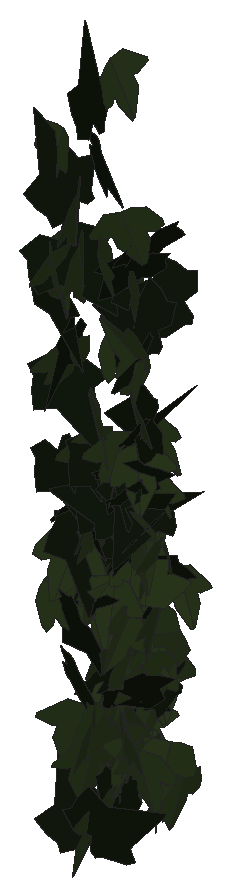
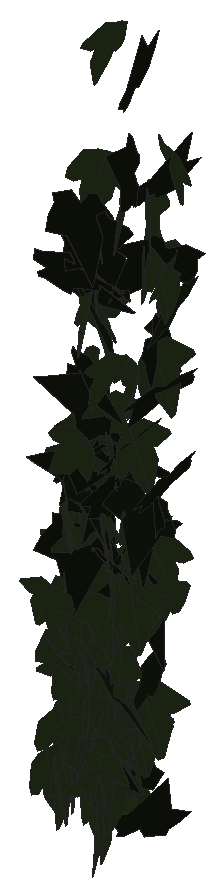
# SketchUp Ruby script. Lengths in inches.
U = 1.inch
M = Sketchup.active_model
def pt(a) = Geom::Point3d.new(a.map { |v| v * U })
def face(e, loops, mat)
  f = e.add_face(loops[0].map { |a| pt(a) })
  loops[1..].each { |l| e.add_face(l.map { |a| pt(a) }).erase! }
  f.material = f.back_material = mat if mat
  f
end
# faces: each face lists its corners as indices into pts; further lists are holes
def faces(e, pts, list, mat = nil) = list.each { |f| face(e, (f[0].is_a?(Array) ? f : [f]).map { |l| l.map { |i| pts[i] } }, mat) }
# xy, xz, yz: faces in a plane at the given z, y or x. An outline is a flat list of corners, or four numbers for a rectangle; further outlines are holes
def ring(l) = l.size == 4 ? [[l[0], l[1]], [l[2], l[1]], [l[2], l[3]], [l[0], l[3]]] : l.each_slice(2).to_a
def flat(e, list, mat, &to3) = list.each { |f| face(e, (f[0].is_a?(Array) ? f : [f]).map { |l| ring(l).map { |u, v| to3.(u, v) } }, mat) }
def xy(e, z, list, mat = nil) = flat(e, list, mat) { |x, y| [x, y, z] }
def xz(e, y, list, mat = nil) = flat(e, list, mat) { |x, z| [x, y, z] }
def yz(e, x, list, mat = nil) = flat(e, list, mat) { |y, z| [x, y, z] }
def lines(e, pts, list) = list.each { |a, b| e.add_line(pt(pts[a]), pt(pts[b])) }
# prism: a flat outline (further loops are holes) pulled along v
def prism(e, loops, v, mat = nil)
  f = face(e, loops, mat); d = Geom::Vector3d.new(v.map { |x| x * U })
  f.pushpull(f.normal.samedirection?(d) ? d.length : -d.length)
end
def box(e, o, s, mat = nil) = prism(e, [[o, [o[0] + s[0], o[1], o[2]], [o[0] + s[0], o[1] + s[1], o[2]], [o[0], o[1] + s[1], o[2]]]], [0, 0, s[2]], mat)
def at(x, y, z, deg = 0) = Geom::Transformation.translation(pt([x, y, z])) * Geom::Transformation.rotation(ORIGIN, Z_AXIS, deg.degrees)
def axes(o, x, y, z) = Geom::Transformation.new([*x, 0, *y, 0, *z, 0, *pt(o).to_a, 1])
def part(name) = M.definitions.add(name)
# library, detail: a bought-in or finely detailed component or shape, given as its bounding box
def library(name, o, s) = part(name).tap { |d| box(d.entities, o, s) }
def detail(e, o, s) = box(e.add_group.entities, o, s)
def put(e, d, t, mat = nil) = e.add_instance(d, t).tap { |i| i.material = mat if mat }
def group(e, t, mat = nil) = e.add_group.tap { |g| g.transformation = t; g.material = mat if mat }.entities
root = M.entities
M.materials.add("efeu1").color = [18, 25, 13]
M.materials.add("efeu2").color = [43, 57, 29]
c1 = part("ivyleaf_9")
p = [[1.54,2.16,1.25],[1.36,2.04,1.19],[-0.21,0.99,0.68],[-0.71,1.11,0.82],[-0.85,0.86,0.67],[-0.8,0.17,0.21],
  [-0.9,-0.01,0.1],[-0.67,-0.16,-0.02],[-0.08,-0.08,-0.05],[-0.03,-0.6,-0.4],[0.65,-0.88,-0.66],[0.83,-0.6,-0.49],
  [1.29,-0.42,-0.43],[1.8125,-0.07,-0.26],[1.21,0.44,0.15]]
faces(c1.entities,p,[[0,1,2,3,4,5,6,7,8,9,10,11,12,13,14]],"efeu1")
c2 = part("ivyleaf_10")
p = [[0,0.5,-0.03],[-0.0625,2.02,-0.43],[-0.19,2.01,-0.46],[-0.54,1.05,-0.29],[-0.52,0.625,-0.18],[-0.83,0.76,-0.28],
  [-1.16,0.64,-0.33],[-1.15,0.33,-0.24],[-0.77,-0.39,0.02],[-0.3,-0.51,0.16],[0.04,-0.48,0.23],[-0.02,2.01,-0.4375],
  [-0.06,2.01,-0.43],[0.04,-0.49,0.23],[0.67,-0.49,0.14],[1.38,0.36,-0.2],[1.375,0.51,-0.24],[0.81,0.65,-0.19],
  [0.62,0.59,-0.15],[0.6,1.09,-0.28],[0.5,1.23,-0.31]]
faces(c2.entities,p,[[0,1,2,3,4,5,6,7,8,9,10],[11,12,0,13,14,15,16,17,18,19,20]],"efeu2")
put(root,c1,axes([503.85,135.93,193.72],[0.29247,-0.67636,-0.23949],[-0.06673,0.23186,-0.73631],[0.7144,0.29856,0.02927]))
put(root,c2,axes([504.13,135.48,202.97],[0.65071,-0.36372,0.02117],[0.02149,-0.00643,-0.73192],[0.39285,0.60282,0.00497]))
put(root,c2,axes([504.11,135.52,199.69],[-0.29868,0.74738,-0.07122],[0.01965,-0.06884,-0.80482],[-0.75051,-0.29924,0.00727]))
put(root,c2,axes([504.05,135.49,190.06],[0.08819,0.63214,0.37363],[0.04455,0.35691,-0.66288],[-0.784,0.09138,0.00436]))
put(root,c2,axes([504.33,135.49,199.79],[-0.02818,-0.80038,-0.11798],[-0.0198,0.11869,-0.80053],[0.80879,-0.02498,-0.02371]))
put(root,c2,axes([504.36,135.71,196.93],[-0.09748,-0.77423,0.14032],[-0.03583,-0.13688,-0.78013],[0.78602,-0.10226,-0.01816]))
put(root,c1,axes([503.82,135.64,198.59],[0.40294,-0.67919,0.14319],[0.07626,-0.12125,-0.78971],[0.68992,0.41008,0.00366]))
put(root,c1,axes([504.55,136.12,183.22],[-0.54458,-0.44797,0.2202],[0.19318,0.11714,0.70079],[-0.49904,0.5342,0.03098]))
put(root,c2,axes([504.46,136.59,190.1875],[-0.26662,-0.69959,0.04964],[0.01187,-0.0576,-0.74801],[0.70125,-0.26501,0.03153]))
put(root,c1,axes([504.57,135.91,192.6875],[0.16065,0.67425,0.16954],[-0.05888,0.17758,-0.71209],[-0.74686,0.13103,0.09261]))
put(root,c1,axes([504.06,135.82,196.26],[0.19336,-0.71103,-0.28018],[0.06705,0.30368,-0.72439],[0.7613,0.15385,0.13496]))
put(root,c1,axes([504.7,135.33,201.68],[-0.32899,-0.68329,0.30857],[0.1248,0.28235,0.75831],[-0.73928,0.35174,-0.0093]))
put(root,c2,axes([504.45,135.7,191.39],[0.73109,0.20015,-0.15467],[-0.15667,-0.03386,-0.73409],[-0.21904,0.69226,0.00881]))
put(root,c1,axes([504.35,135.73,187.875],[0.57329,-0.21264,-0.36386],[-0.32972,0.17613,-0.59305],[0.29463,0.61087,0.04433]))
put(root,c1,axes([504.71,135.71,192.4],[0.42549,0.08154,-0.57527],[-0.60291,0.01959,-0.41051],[-0.03371,0.67882,0.08095]))
put(root,c2,axes([504.79,135.7,186.67],[-0.54553,-0.51842,0.24353],[-0.14596,-0.19939,-0.7514],[0.55386,-0.56316,0.04185]))
put(root,c1,axes([504.49,135.67,197.51],[-0.20411,0.17828,-0.66152],[0.50675,-0.42947,-0.27017],[-0.50219,-0.50583,-0.00376]))
put(root,c1,axes([505.07,136.51,185.14],[-0.17766,0.29629,0.61295],[-0.30257,0.51855,-0.35243],[-0.645,-0.32486,-0.00351]))
put(root,c1,axes([504.26,135.5,200.09],[0.00591,-0.44392,-0.67778],[0.222,0.65274,-0.42559],[0.77921,-0.1826,0.1264]))
put(root,c1,axes([505.06,136.83,187.7],[-0.53617,0.43246,0.0549],[-0.04682,0.0306,-0.68471],[-0.46819,-0.49832,0.0056]))
put(root,c2,axes([504.64,136,191.47],[0.23655,-0.57216,0.31831],[-0.12167,0.2846,0.63715],[-0.69014,-0.24629,-0.00323]))
put(root,c2,axes([504.72,136.72,188.32],[0.11736,-0.65889,-0.32619],[0.00512,0.33104,-0.66685],[0.7352,0.10287,0.05671]))
put(root,c2,axes([504.79,136.9,184.89],[-0.09356,-0.66841,-0.24276],[0.04432,0.2389,-0.67485],[0.70975,-0.10303,0.01014]))
put(root,c2,axes([504.8,135.375,201.47],[0.27227,-0.72391,-0.265],[-0.0089,0.27807,-0.76877],[0.77084,0.25891,0.08472]))
put(root,c1,axes([504.52,136.09,191.7],[0.01968,-0.76216,-0.05621],[-0.00299,0.05615,-0.76241],[0.76423,0.01985,-0.00153]))
put(root,c2,axes([504.83,136.62,190.23],[0.14349,-0.65581,-0.33627],[0.01404,0.34496,-0.66675],[0.73686,0.12114,0.07819]))
put(root,c1,axes([505.2,135.09,189.75],[0.25131,0.19547,-0.76499],[-0.777,-0.08144,-0.27606],[-0.14031,0.80108,0.1586]))
put(root,c2,axes([504.84,136.6,190.38],[0.1255,-0.71483,-0.19602],[0.00745,0.20002,-0.72463],[0.74118,0.11903,0.04047]))
put(root,c2,axes([504.9,135.97,194.43],[-0.08873,-0.75427,0.18352],[0.0204,-0.18692,-0.75836],[0.776,-0.08133,0.04092]))
put(root,c2,axes([504.96,137.09,184.1],[0.14571,-0.58366,-0.38437],[-0.06892,0.37872,-0.60121],[0.69545,0.15982,0.02095]))
put(root,c2,axes([504.9,137.43,183.88],[0.3272,-0.56485,-0.26269],[0.036,0.31337,-0.62898],[0.6219,0.27904,0.17461]))
put(root,c2,axes([504.99,136.02,192.12],[0.13697,-0.67875,-0.32838],[0.03072,0.3385,-0.68686],[0.75339,0.10959,0.08771]))
put(root,c2,axes([505.01,135.22,200.06],[0.27493,-0.71871,-0.2534],[0.07213,0.29272,-0.75197],[0.75866,0.23262,0.16333]))
put(root,c2,axes([505.16,135.59,185.85],[-0.22808,-0.69401,0.0999],[-0.0223,-0.09782,-0.73047],[0.70081,-0.22898,0.00927]))
put(root,c2,axes([505.05,137.21,184.8125],[0.45925,-0.54338,-0.06754],[0.00247,0.09021,-0.70894],[0.54755,0.45534,0.05985]))
put(root,c2,axes([505.23,135.43,186.54],[0.20366,-0.64066,-0.42388],[-0.0688,0.42155,-0.67019],[0.7651,0.20844,0.05256]))
put(root,c1,axes([505.59,136.39,190.89],[-0.71501,0.20383,0.05754],[-0.06368,-0.00355,-0.7201],[-0.21904,-0.66435,0.0215]))
put(root,c2,axes([505.08,137.16,184.9375],[0.2397,0.67519,0.06414],[-0.02972,0.07841,-0.71444],[-0.67758,0.23542,0.05402]))
put(root,c2,axes([505.07,136.6,196.92],[0.0239,0.5762,0.30791],[0.02519,0.29534,-0.59958],[-0.69918,0.03033,-0.01108]))
put(root,c2,axes([505.01,136.88,186.875],[0.61212,0.3818,0.10176],[0.06428,0.08892,-0.72027],[-0.38987,0.61412,0.04102]))
put(root,c2,axes([505.37,136.98,185.8125],[-0.18151,-0.41509,0.5609],[-0.11951,-0.55251,-0.44755],[0.68747,-0.20564,0.07029]))
put(root,c2,axes([505.04,137.17,185.39],[0.65485,0.27704,0.11574],[0.09951,0.06173,-0.71082],[-0.28327,0.66213,0.01785]))
put(root,c1,axes([504.72,136.26,202.5625],[0.19608,-0.05369,-0.67659],[0.70177,-0.04966,0.19285],[-0.06736,-0.6736,0.03972]))
put(root,c2,axes([505.24,135.73,183.92],[0.21221,-0.65109,0.3794],[0.09858,-0.36678,-0.68457],[0.74709,0.23334,-0.01744]))
put(root,c2,axes([505.32,137.26,184.47],[0.14229,-0.6955,0.01762],[0.02136,-0.01361,-0.70967],[0.6954,0.14273,0.01819]))
put(root,c2,axes([505.38,137.17,184.2],[0.4199,-0.55474,-0.16486],[-0.05463,0.16478,-0.69361],[0.57613,0.41993,0.05439]))
put(root,c1,axes([505.05,135.88,194.29],[0.25686,-0.70449,-0.20401],[-0.02539,0.20749,-0.74847],[0.733,0.25406,0.04556]))
put(root,c2,axes([505.41,136.75,187.11],[-0.34813,-0.62884,-0.16639],[0.10716,0.13069,-0.71816],[0.64159,-0.36304,0.02967]))
put(root,c1,axes([505.61,135.05,204.34],[-0.10083,-0.50517,0.65479],[0.13692,0.64033,0.5151],[-0.81559,0.16995,0.00552]))
put(root,c2,axes([505.43,137.02,185.69],[0.68319,0.19789,-0.13654],[-0.13545,-0.023,-0.71111],[-0.19864,0.69632,0.01531]))
put(root,c2,axes([505.41,136.69,189.56],[-0.72112,-0.02035,-0.16316],[0.16434,-0.06539,-0.71817],[0.00534,-0.73645,0.06828]))
put(root,c1,axes([505.21,136.13,193.21],[0.17575,-0.63052,-0.48216],[-0.08503,0.47604,-0.65351],[0.78918,0.19171,0.03696]))
put(root,c2,axes([505.49,136.45,191.8],[0.39405,-0.64188,-0.09922],[0.01309,0.12387,-0.74941],[0.64937,0.38701,0.07531]))
put(root,c2,axes([505.42,135.42,195.79],[-0.49829,0.56556,-0.12774],[0.05894,-0.11386,-0.75847],[-0.62226,-0.46367,0.03045]))
put(root,c2,axes([505.68,136.96,198.64],[-0.41799,0.36555,0.34872],[-0.24734,0.24557,-0.55335],[-0.47521,-0.44935,-0.01872]))
put(root,c2,axes([505.6,136.0625,194.02],[0.45016,-0.63597,-0.24936],[-0.08748,0.2425,-0.77641],[0.67748,0.45389,0.06543]))
put(root,c2,axes([505.52,136.5,186.58],[-0.42623,0.61962,0.01152],[-0.00791,0.00855,-0.75207],[-0.61968,-0.4263,0.00167]))
put(root,c2,axes([505.58,136.47,186.91],[-0.00479,-0.64637,-0.35972],[0.09243,0.35638,-0.6416],[0.73392,-0.0491,0.07846]))
put(root,c2,axes([506.09,136.98,185.37],[-0.01324,0.02492,-0.63066],[-0.65496,0.02342,0.01375],[0.02586,0.60608,0.0254]))
put(root,c2,axes([505.67,136.17,184.63],[-0.04849,-0.71919,-0.11963],[0.02509,0.11817,-0.72062],[0.72864,-0.05193,0.01685]))
put(root,c1,axes([506.09,135.67,184.37],[-0.07312,0.16088,0.66524],[-0.4149,0.51307,-0.1765],[-0.57904,-0.38794,0.04246]))
put(root,c2,axes([505.8125,135.97,190.22],[-0.45941,-0.51113,0.3166],[-0.09837,-0.32918,-0.67418],[0.59314,-0.45048,0.13341]))
put(root,c2,axes([505.75,135.9,185.09],[0.45415,-0.45244,-0.34408],[-0.10902,0.36291,-0.62109],[0.55787,0.43925,0.15874]))
put(root,c1,axes([506.32,135.36,193.32],[-0.43687,0.13189,0.5506],[-0.5481,0.15102,-0.4424],[-0.21634,-0.64893,0.00896]))
put(root,c2,axes([505.42,136.5625,184.09],[-0.2791,0.20552,-0.62921],[0.33724,-0.54344,-0.32709],[-0.56958,-0.42247,0.11465]))
put(root,c2,axes([505.72,135.55,187.01],[-0.03496,-0.55942,-0.56628],[0.12688,0.55567,-0.55677],[0.78583,-0.1146,0.0647]))
put(root,c2,axes([505.54,136.92,186.24],[0.30527,0.61406,0.24078],[0.11036,0.21402,-0.68575],[-0.65028,0.32459,-0.00335]))
put(root,c2,axes([505.78,136.7,187.88],[0.32467,-0.62627,-0.21445],[0.01632,0.24636,-0.69473],[0.66176,0.30118,0.12235]))
put(root,c2,axes([505.87,136.1875,188.24],[-0.00982,0.65143,-0.34534],[-0.1261,-0.34176,-0.6411],[-0.72644,0.05052,0.11596]))
put(root,c2,axes([505.76,135.63,190.57],[0.75117,0.04653,0.05442],[0.05644,0.00271,-0.72496],[-0.05033,0.69749,-0.00082]))
put(root,c2,axes([506.16,134.83,200.61],[-0.31516,0.34436,0.57995],[-0.38705,0.42724,-0.46943],[-0.59264,-0.46216,-0.00183]))
put(root,c2,axes([506.03,135.81,194.82],[-0.2352,-0.71325,0.21046],[0.03082,-0.2299,-0.74467],[0.74302,-0.21624,0.09751]))
put(root,c1,axes([505.48,135.84,189.7],[0.45841,0.51038,-0.29116],[0.19831,0.2114,0.69034],[0.59659,-0.46243,-0.00576]))
put(root,c2,axes([506.2,136.34,185.92],[-0.33057,-0.51756,0.37757],[-0.11574,-0.36963,-0.60801],[0.6301,-0.33943,0.0864]))
put(root,c2,axes([505.79,137.22,194.57],[-0.54807,0.09603,-0.36211],[0.35706,-0.11826,-0.53506],[-0.15706,-0.60396,0.04719]))
put(root,c1,axes([506.33,135.91,200.11],[-0.03529,0.51555,-0.43584],[-0.11499,-0.41822,-0.52644],[-0.70827,0.04222,0.10719]))
put(root,c2,axes([506.13,136.65,189.3125],[0.04219,-0.74568,-0.04214],[-0.02226,0.04093,-0.74661],[0.74654,0.04336,-0.01988]))
put(root,c2,axes([506.2,136.85,187.7],[-0.22723,-0.68618,0.13756],[0.00233,-0.14537,-0.72129],[0.69983,-0.22232,0.04707]))
put(root,c1,axes([505.54,135.24,183.73],[0.03066,0.00418,0.77404],[0.76419,-0.23115,-0.02672],[0.2493,0.70804,-0.0133]))
put(root,c2,axes([506.21,136.42,185.84],[-0.00636,-0.72143,0.06981],[0.01159,-0.0699,-0.72136],[0.72471,-0.00521,0.01215]))
put(root,c2,axes([506.5,135.34,186.8],[-0.53675,0.29759,0.43417],[-0.40229,0.1899,-0.60196],[-0.38044,-0.62066,0.02399]))
put(root,c1,axes([506.04,135.62,194.05],[0.62697,0.43726,0.04484],[0.04109,0.02115,-0.75582],[-0.47274,0.58174,-0.00623]))
put(root,c1,axes([506.59,136.02,192.86],[-0.3524,0.62619,-0.00527],[-0.00076,-0.00608,-0.73434],[-0.67631,-0.32628,0.00357]))
put(root,c2,axes([506.16,136.23,191.34],[0.40397,0.59229,-0.01092],[-0.03823,0.00995,-0.72761],[-0.63863,0.37406,0.03665]))
put(root,c2,axes([506.09,136.92,187.88],[0.40445,0.53869,0.12196],[0.06866,0.09862,-0.6823],[-0.59144,0.37982,0.00419]))
put(root,c2,axes([506.21,135.28,205.76],[0.02047,0.65963,0.23119],[-0.04349,0.22305,-0.68475],[-0.7505,0.00507,0.04599]))
put(root,c2,axes([505.85,136.12,186.61],[-0.32135,0.1225,0.6471],[0.63368,-0.2076,0.33431],[0.25986,0.65771,-0.015]))
put(root,c1,axes([506.72,135.36,197.59],[-0.27205,0.51536,0.44697],[-0.18347,0.39513,-0.59632],[-0.70113,-0.30337,-0.01739]))
put(root,c2,axes([506.22,135.6,192.8125],[-0.69642,0.09075,-0.15531],[0.16032,-0.01673,-0.67722],[-0.09956,-0.66169,-0.00417]))
put(root,c2,axes([506.33,137.28,184.78],[0.27431,-0.65072,-0.08738],[-0.00663,0.09195,-0.70556],[0.65653,0.27282,0.02939]))
put(root,c1,axes([506.36,136.26,191.3],[0.44813,0.51501,-0.25104],[-0.16885,-0.18401,-0.6878],[-0.59062,0.44337,0.00615]))
put(root,c2,axes([506.83,135.33,197.66],[-0.28483,0.11628,-0.67175],[-0.62971,0.27802,0.29965],[0.32536,0.63989,-0.00812]))
put(root,c2,axes([506.3125,136.73,187.4],[-0.10406,-0.64422,0.33473],[0.1105,-0.34827,-0.63592],[0.71753,-0.0398,0.14648]))
put(root,c2,axes([506.32,135.61,189.89],[0.06295,0.45616,-0.49069],[-0.12381,-0.45932,-0.47657],[-0.69788,0.12263,0.04028]))
put(root,c2,axes([505.8125,136.51,188.28],[-0.02633,-0.05459,-0.65142],[0.61743,-0.2628,0.00067],[-0.2826,-0.56908,0.06218]))
put(root,c2,axes([506.46,136.51,184.79],[0.39782,-0.38453,-0.4634],[-0.14921,0.47513,-0.52235],[0.58339,0.38373,0.1824]))
put(root,c1,axes([506.9,135.8,195.8],[-0.15858,0.01324,-0.70381],[-0.71831,-0.13142,0.14741],[-0.13576,0.67991,0.0422]))
put(root,c2,axes([506.38,137.08,184.625],[0.0882,-0.67555,-0.229],[0.0378,0.23485,-0.67824],[0.7123,0.07119,0.06435]))
put(root,c2,axes([506.35,136.82,188.29],[0.68777,-0.19714,-0.07209],[-0.06773,0.03178,-0.6932],[0.21529,0.6398,0.01222]))
put(root,c2,axes([506.49,136.71,188.34],[-0.58694,-0.44455,0.0232],[-0.01864,-0.01382,-0.73629],[0.44476,-0.58724,-0.00024]))
put(root,c2,axes([506.9,136.66,189.4],[-0.33649,0.00305,0.66554],[-0.66089,-0.08967,-0.33372],[0.07866,-0.74036,0.04316]))
put(root,c1,axes([506.98,135.86,198.43],[-0.40496,0.217,0.54901],[-0.49013,0.26969,-0.45054],[-0.37382,-0.58867,-0.00403]))
put(root,c1,axes([506.7,135.51,192.43],[-0.26054,0.68249,-0.13222],[0.05683,-0.11623,-0.75275],[-0.74762,-0.24668,-0.01114]))
put(root,c1,axes([506.85,136.71,187.96],[-0.63591,0.32074,0.02412],[-0.05508,-0.04537,-0.69412],[-0.34291,-0.58751,0.06677]))
put(root,c2,axes([506.61,135.6,196.05],[-0.53959,0.42621,0.25886],[-0.2119,0.15347,-0.6829],[-0.48912,-0.53667,0.01028]))
put(root,c1,axes([506.68,135.95,200.76],[-0.00053,0.668,-0.16644],[0.00594,-0.16003,-0.6947],[-0.74183,-0.00176,-0.00545]))
put(root,c1,axes([506.28,135.75,195.01],[-0.05791,0.684,-0.2356],[-0.02282,0.22557,0.71354],[0.77785,0.05754,0.00339]))
put(root,c2,axes([506.85,136.43,192.02],[-0.24724,0.22538,0.55434],[-0.50595,0.26436,-0.3255],[-0.36694,-0.51636,0.07531]))
put(root,c2,axes([506.6,136.41,190.02],[0.225,-0.71379,-0.01859],[0.00428,0.02085,-0.74834],[0.71402,0.2248,0.01035]))
put(root,c1,axes([506.5,136.17,193.375],[-0.31381,-0.67981,0.19343],[-0.00454,-0.2097,-0.74434],[0.70678,-0.30318,0.08111]))
put(root,c2,axes([506.3,137.67,190.22],[0.55955,0.14685,0.25657],[0.25347,0.07653,-0.55997],[-0.17859,0.56871,0.0091]))
put(root,c2,axes([506.73,135.34,199.36],[0.43934,-0.54122,-0.47949],[-0.17366,0.46566,-0.68473],[0.7019,0.45398,0.13071]))
put(root,c2,axes([506.49,135.77,194.55],[0.34172,0.60851,-0.01526],[-0.00739,-0.01298,-0.71329],[-0.65734,0.31648,0.00008]))
put(root,c2,axes([506.8,135.35,197.64],[0.46187,-0.45647,-0.35331],[-0.24942,0.24916,-0.65052],[0.56164,0.48603,0.00166]))
put(root,c2,axes([506.6,135.19,201.69],[-0.56794,-0.4255,-0.18879],[0.16033,0.10508,-0.70341],[0.47319,-0.54631,0.01175]))
put(root,c1,axes([506.51,135.27,188.22],[0.45575,0.50161,0.13859],[0.08968,0.10429,-0.68172],[-0.55331,0.43007,0.00367]))
put(root,c2,axes([506.63,135.79,185.93],[-0.74859,-0.01122,-0.09197],[0.09609,-0.04554,-0.71933],[0.00577,-0.69728,0.04846]))
put(root,c2,axes([506.35,136.3,193.5],[0.68959,0.17764,0.2602],[0.23258,0.13536,-0.70878],[-0.21253,0.72451,0.06863]))
put(root,c2,axes([506.58,136.05,190.76],[0.74021,0.21742,-0.00704],[0.00366,0.01251,0.7714],[0.2175,-0.74014,0.01097]))
put(root,c2,axes([506.74,136.67,185.82],[-0.45799,-0.52435,0.20699],[0.02783,-0.2874,-0.66646],[0.56304,-0.41231,0.20131]))
put(root,c1,axes([507.22,136.5625,199],[-0.51355,0.0658,0.47988],[-0.49723,0.03641,-0.49883],[-0.07844,-0.66159,0.02027]))
put(root,c2,axes([506.74,137.21,184.82],[-0.13215,-0.69695,0.09346],[-0.00106,-0.0949,-0.70918],[0.70319,-0.13112,0.01649]))
put(root,c2,axes([506.69,136.31,191.84],[0.25243,-0.71206,0.1365],[0.0234,-0.13646,-0.75513],[0.72465,0.25245,-0.02317]))
put(root,c2,axes([506.6,135.8125,192.24],[-0.09588,0.64221,-0.07791],[0.00131,-0.07545,-0.67419],[-0.69829,-0.08832,0.00943]))
put(root,c1,axes([506.26,135.61,192.96],[0.24476,0.0577,0.6468],[0.6129,0.25733,-0.2399],[-0.28177,0.60986,0.04003]))
put(root,c2,axes([506.68,135.85,188.5],[-0.26305,-0.61,-0.35285],[0.14345,0.3224,-0.66429],[0.68995,-0.2996,0.00358]))
